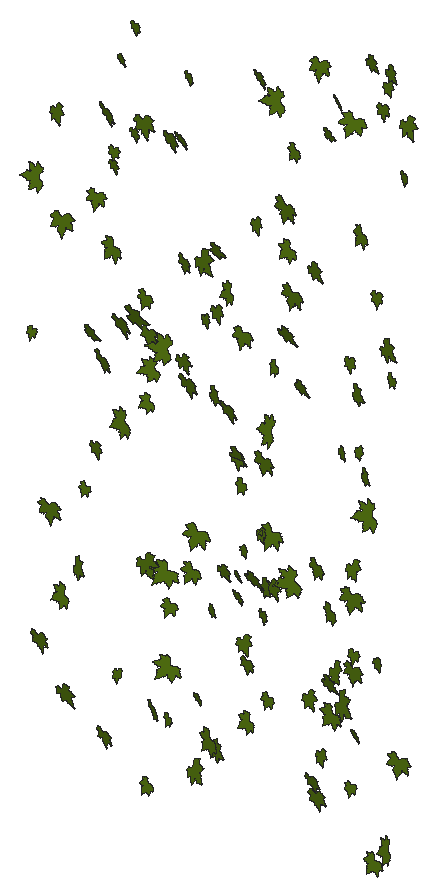
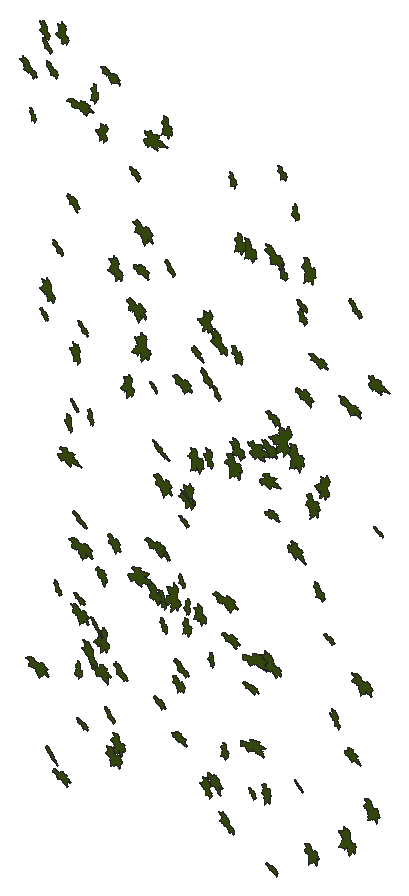
# SketchUp Ruby script. Lengths in inches.
U = 1.inch
M = Sketchup.active_model
def pt(a) = Geom::Point3d.new(a.map { |v| v * U })
def face(e, loops, mat)
  f = e.add_face(loops[0].map { |a| pt(a) })
  loops[1..].each { |l| e.add_face(l.map { |a| pt(a) }).erase! }
  f.material = f.back_material = mat if mat
  f
end
# faces: each face lists its corners as indices into pts; further lists are holes
def faces(e, pts, list, mat = nil) = list.each { |f| face(e, (f[0].is_a?(Array) ? f : [f]).map { |l| l.map { |i| pts[i] } }, mat) }
# xy, xz, yz: faces in a plane at the given z, y or x. An outline is a flat list of corners, or four numbers for a rectangle; further outlines are holes
def ring(l) = l.size == 4 ? [[l[0], l[1]], [l[2], l[1]], [l[2], l[3]], [l[0], l[3]]] : l.each_slice(2).to_a
def flat(e, list, mat, &to3) = list.each { |f| face(e, (f[0].is_a?(Array) ? f : [f]).map { |l| ring(l).map { |u, v| to3.(u, v) } }, mat) }
def xy(e, z, list, mat = nil) = flat(e, list, mat) { |x, y| [x, y, z] }
def xz(e, y, list, mat = nil) = flat(e, list, mat) { |x, z| [x, y, z] }
def yz(e, x, list, mat = nil) = flat(e, list, mat) { |y, z| [x, y, z] }
def lines(e, pts, list) = list.each { |a, b| e.add_line(pt(pts[a]), pt(pts[b])) }
# prism: a flat outline (further loops are holes) pulled along v
def prism(e, loops, v, mat = nil)
  f = face(e, loops, mat); d = Geom::Vector3d.new(v.map { |x| x * U })
  f.pushpull(f.normal.samedirection?(d) ? d.length : -d.length)
end
def box(e, o, s, mat = nil) = prism(e, [[o, [o[0] + s[0], o[1], o[2]], [o[0] + s[0], o[1] + s[1], o[2]], [o[0], o[1] + s[1], o[2]]]], [0, 0, s[2]], mat)
def at(x, y, z, deg = 0) = Geom::Transformation.translation(pt([x, y, z])) * Geom::Transformation.rotation(ORIGIN, Z_AXIS, deg.degrees)
def axes(o, x, y, z) = Geom::Transformation.new([*x, 0, *y, 0, *z, 0, *pt(o).to_a, 1])
def part(name) = M.definitions.add(name)
# library, detail: a bought-in or finely detailed component or shape, given as its bounding box
def library(name, o, s) = part(name).tap { |d| box(d.entities, o, s) }
def detail(e, o, s) = box(e.add_group.entities, o, s)
def put(e, d, t, mat = nil) = e.add_instance(d, t).tap { |i| i.material = mat if mat }
def group(e, t, mat = nil) = e.add_group.tap { |g| g.transformation = t; g.material = mat if mat }.entities
root = M.entities
M.materials.add("[Vegetation Blur 03]").color = [83, 114, 18]
c1 = part("ivy")
xy(c1.entities,0,[[0.782,0,0.786,0,0.787,0.005,0.789,0.009,0.821,0.072,0.875,0.147,1.001,0.272,1.073,0.331,1.137,0.363,1.178,0.379,1.223,0.384,1.272,0.383,1.311,0.374,1.36,0.355,1.399,0.334,1.491,0.285,1.541,0.244,1.583,0.199,1.617,0.15,1.64,0.128,1.662,0.115,1.717,0.105,1.745,0.093,1.784,0.054,1.819,0.057,1.854,0.064,1.882,0.075,1.896,0.074,1.91,0.071,1.937,0.063,1.964,0.053,1.99,0.038,2.016,0.015,2.034,0.002,2.04,0,2.038,0.003,2.036,0.007,2.033,0.038,2.036,0.068,2.045,0.1,2.055,0.116,2.064,0.123,2.077,0.129,2.088,0.129,2.106,0.132,2.118,0.13,2.179,0.132,2.207,0.133,2.225,0.133,2.242,0.138,2.22,0.162,2.207,0.186,2.206,0.213,2.212,0.236,2.228,0.262,2.247,0.274,2.298,0.283,2.355,0.294,2.37,0.296,2.376,0.295,2.377,0.3,2.377,0.303,2.385,0.329,2.411,0.37,2.426,0.392,2.449,0.407,2.511,0.426,2.561,0.444,2.619,0.466,2.589,0.469,2.561,0.476,2.501,0.5,2.449,0.516,2.424,0.523,2.401,0.535,2.377,0.556,2.372,0.568,2.36,0.575,2.268,0.586,2.225,0.592,2.207,0.599,2.194,0.61,2.143,0.65,2.13,0.664,2.122,0.682,2.123,0.7,2.13,0.719,2.148,0.75,2.17,0.781,2.195,0.807,2.221,0.828,2.284,0.874,2.291,0.88,2.288,0.887,2.276,0.9,2.267,0.916,2.265,0.933,2.273,0.967,2.292,1.002,2.313,1.03,2.334,1.054,2.348,1.067,2.358,1.074,2.363,1.076,2.362,1.081,2.35,1.094,2.347,1.11,2.35,1.143,2.359,1.18,2.385,1.254,2.415,1.324,2.448,1.393,2.45,1.4,2.446,1.398,2.44,1.394,2.427,1.383,2.402,1.36,2.376,1.339,2.345,1.324,2.305,1.309,2.282,1.303,2.273,1.306,2.245,1.294,2.212,1.287,2.187,1.291,2.163,1.301,2.142,1.316,2.134,1.327,2.124,1.325,2.09,1.292,2.053,1.259,2.014,1.234,1.973,1.215,1.954,1.21,1.931,1.208,1.909,1.212,1.893,1.22,1.879,1.233,1.872,1.248,1.867,1.281,1.864,1.319,1.821,1.258,1.773,1.197,1.726,1.141,1.698,1.121,1.679,1.116,1.666,1.117,1.647,1.122,1.632,1.129,1.62,1.141,1.617,1.154,1.617,1.219,1.621,1.254,1.623,1.268,1.623,1.281,1.618,1.314,1.606,1.346,1.603,1.375,1.607,1.403,1.603,1.467,1.599,1.499,1.605,1.525,1.614,1.552,1.629,1.577,1.635,1.589,1.629,1.587,1.618,1.582,1.596,1.566,1.581,1.556,1.568,1.552,1.557,1.55,1.545,1.553,1.531,1.562,1.522,1.572,1.504,1.591,1.486,1.611,1.474,1.631,1.457,1.666,1.455,1.684,1.457,1.698,1.452,1.715,1.444,1.728,1.424,1.754,1.419,1.772,1.423,1.786,1.434,1.819,1.444,1.848,1.446,1.855,1.44,1.861,1.43,1.867,1.386,1.904,1.349,1.948,1.326,1.973,1.31,1.995,1.288,2.048,1.284,2.153,1.287,2.254,1.284,2.255,1.282,2.253,1.278,2.247,1.274,2.237,1.266,2.216,1.226,2.125,1.208,2.076,1.184,2.033,1.155,1.984,1.135,1.942,1.111,1.899,1.083,1.861,1.053,1.85,1.059,1.83,1.061,1.809,1.056,1.79,1.049,1.767,1.04,1.749,1.018,1.733,0.994,1.726,0.942,1.734,0.95,1.6875,0.944,1.645,0.932,1.608,0.911,1.585,0.881,1.58,0.854,1.582,0.828,1.588,0.785,1.618,0.773,1.625,0.775,1.614,0.779,1.598,0.796,1.502,0.818,1.402,0.861,1.283,0.882,1.224,0.894,1.174,0.892,1.148,0.886,1.123,0.881,1.107,0.872,1.099,0.849,1.094,0.818,1.092,0.789,1.098,0.762,1.107,0.753,1.113,0.721,1.139,0.698,1.163,0.678,1.194,0.665,1.224,0.628,1.28,0.612,1.312,0.606,1.327,0.606,1.314,0.599,1.282,0.594,1.267,0.581,1.256,0.544,1.245,0.512,1.244,0.473,1.249,0.444,1.256,0.382,1.288,0.339,1.306,0.324,1.316,0.317,1.324,0.309,1.326,0.27,1.314,0.227,1.313,0.185,1.3125,0.152,1.317,0.122,1.328,0.092,1.345,0.073,1.353,0.079,1.338,0.092,1.308,0.117,1.249,0.13,1.215,0.139,1.164,0.147,1.148,0.157,1.136,0.163,1.122,0.174,1.086,0.177,1.067,0.182,1.054,0.186,1.043,0.191,1.038,0.211,1.028,0.237,1.005,0.25,0.974,0.253,0.96,0.25,0.944,0.242,0.914,0.243,0.906,0.249,0.902,0.26,0.894,0.289,0.88,0.307,0.873,0.322,0.862,0.364,0.799,0.403,0.738,0.431,0.709,0.439,0.691,0.441,0.678,0.4375,0.66,0.428,0.645,0.394,0.623,0.303,0.594,0.255,0.581,0.214,0.577,0.179,0.573,0.173,0.568,0.175,0.561,0.167,0.55,0.141,0.523,0.113,0.503,0.077,0.49,0.045,0.486,0.026,0.485,0.019,0.486,0.011,0.483,0,0.471,0.014,0.467,0.044,0.455,0.058,0.447,0.07,0.438,0.097,0.411,0.125,0.394,0.158,0.377,0.174,0.366,0.182,0.359,0.185,0.361,0.242,0.331,0.253,0.316,0.258,0.303,0.262,0.283,0.274,0.278,0.308,0.274,0.341,0.252,0.366,0.226,0.366,0.222,0.37,0.22,0.38,0.221,0.395,0.221,0.425,0.216,0.45,0.207,0.465,0.192,0.473,0.178,0.484,0.15,0.489,0.116,0.483,0.089,0.468,0.058,0.45,0.035,0.435,0.018,0.429,0.011,0.434,0.012,0.438,0.014,0.469,0.019,0.542,0.016,0.581,0.015,0.612,0.027,0.68,0.055,0.696,0.057,0.712,0.052,0.73,0.045,0.741,0.036,0.766,0.014]])
put(root,c1,axes([28.89,173.7,27.51],[0.18332,-0.13201,0.23981],[0.28131,-0.17522,-0.15841],[-0.10639,-0.6908,-0.00565]),"[Vegetation Blur 03]")
put(root,c1,axes([24.48,173.7,22.26],[0.59751,-0.1415,-0.08723],[-0.11552,-0.16395,-0.48523],[-0.05298,-1.23827,0.07421]),"[Vegetation Blur 03]")
put(root,c1,axes([30.97,173.7,25.6875],[0.30037,-0.23448,-0.48095],[-0.59958,-0.05449,-0.24524],[-0.02777,-1.36002,0.09275]),"[Vegetation Blur 03]")
put(root,c1,axes([14.65,173.7,41.15],[0.5598,-0.34639,0.09978],[0.13771,0.07562,-0.47332],[-0.15594,-1.17668,-0.05979]),"[Vegetation Blur 03]")
put(root,c1,axes([11.74,173.7,39.72],[0.34108,-0.07651,0.26436],[0.30846,-0.23678,-0.27587],[-0.10562,-0.93855,0.04805]),"[Vegetation Blur 03]")
put(root,c1,axes([32.59,173.7,43.74],[0.30667,-0.21087,0.08542],[0.09735,-0.07998,-0.26385],[-0.10945,-0.662,0.00467]),"[Vegetation Blur 03]")
put(root,c1,axes([23.32,173.7,18.92],[0.32867,-0.28906,0.36046],[0.45664,0.0115,-0.27589],[-0.07923,-1.13284,-0.09478]),"[Vegetation Blur 03]")
put(root,c1,axes([31.88,173.7,8.15],[0.33567,-0.36714,-0.32626],[-0.40941,0.10373,-0.29893],[-0.15499,-1.06915,0.08303]),"[Vegetation Blur 03]")
put(root,c1,axes([23.83,173.7,46.01],[0.40968,-0.27629,0.16507],[0.21084,0.00024,-0.34848],[-0.12034,-0.94019,-0.0486]),"[Vegetation Blur 03]")
put(root,c1,axes([13.91,173.7,28.49],[0.13916,-0.21976,0.37305],[0.46529,-0.06512,-0.12164],[-0.06205,-0.98109,-0.07549]),"[Vegetation Blur 03]")
put(root,c1,axes([30.85,173.7,36.73],[0.36627,-0.13941,0.12421],[0.13945,-0.15724,-0.30166],[-0.09113,-0.8009,0.0376]),"[Vegetation Blur 03]")
put(root,c1,axes([17.4,173.7,6.27],[0.36884,-0.18268,-0.08765],[-0.12074,-0.10682,-0.30338],[-0.06956,-0.78327,0.06182]),"[Vegetation Blur 03]")
put(root,c1,axes([15.55,173.7,11.24],[0.27201,-0.08351,0.1346],[0.14493,-0.22002,-0.21655],[-0.08857,-0.61651,0.05905]),"[Vegetation Blur 03]")
put(root,c1,axes([28.28,173.7,15.51],[0.22572,0.02556,0.3673],[0.42622,-0.34586,-0.17068],[-0.14503,-0.97663,0.07006]),"[Vegetation Blur 03]")
put(root,c1,axes([12.04,173.7,9.01],[0.44693,-0.21309,0.34937],[0.42945,-0.06761,-0.37241],[-0.09772,-1.27172,-0.03874]),"[Vegetation Blur 03]")
put(root,c1,axes([30.04,173.7,40.08],[0.46163,-0.2581,-0.13642],[-0.17424,-0.01487,-0.3883],[-0.11538,-1.01019,0.04057]),"[Vegetation Blur 03]")
put(root,c1,axes([30.25,173.7,26.5625],[0.11578,-0.07742,0.31422],[0.36947,-0.22297,-0.09932],[-0.11465,-0.79672,-0.00274]),"[Vegetation Blur 03]")
put(root,c1,axes([21.27,173.7,32.5],[0.35673,-0.12377,0.22075],[0.25958,-0.16822,-0.29423],[-0.09696,-0.90576,0.02448]),"[Vegetation Blur 03]")
put(root,c1,axes([11.84,173.7,34.33],[0.60257,-0.08021,0.1387],[0.16152,-0.21723,-0.48713],[-0.06569,-1.26991,0.07457]),"[Vegetation Blur 03]")
put(root,c1,axes([22.43,173.7,24.94],[0.20255,-0.18759,0.41357],[0.50926,-0.09194,-0.17269],[-0.07578,-1.11921,-0.05513]),"[Vegetation Blur 03]")
put(root,c1,axes([16.46,173.7,30.02],[0.0827,-0.23642,0.52033],[0.64705,-0.03418,-0.07095],[-0.03151,-1.3225,-0.09118]),"[Vegetation Blur 03]")
put(root,c1,axes([25.04,173.7,31.12],[0.30532,-0.22387,-0.07925],[-0.10993,-0.04866,-0.26046],[-0.09582,-0.65751,0.04626]),"[Vegetation Blur 03]")
put(root,c1,axes([23.67,173.7,37.91],[0.28926,-0.09005,0.2261],[0.2622,-0.20395,-0.23621],[-0.09958,-0.79857,0.03483]),"[Vegetation Blur 03]")
put(root,c1,axes([23,173.7,24.12],[0.34373,-0.18323,-0.04475],[-0.06771,-0.09451,-0.28552],[-0.07969,-0.71,0.04955]),"[Vegetation Blur 03]")
put(root,c1,axes([14.1,173.7,22.84],[0.37427,-0.16845,0.18276],[0.21743,-0.11081,-0.31265],[-0.09784,-0.89065,0.00433]),"[Vegetation Blur 03]")
put(root,c1,axes([27.89,173.7,14.87],[0.2552,-0.21443,0.36363],[0.45118,-0.05704,-0.2162],[-0.07626,-1.05507,-0.06222]),"[Vegetation Blur 03]")
put(root,c1,axes([24.18,173.7,17.51],[0.3306,-0.20851,0.08999],[0.10594,-0.063,-0.2822],[-0.10584,-0.71438,-0.00138]),"[Vegetation Blur 03]")
put(root,c1,axes([19.09,173.7,30.18],[0.08303,-0.1967,-0.5076],[-0.62878,-0.07669,-0.06383],[0.02474,-1.28895,0.08126]),"[Vegetation Blur 03]")
put(root,c1,axes([19.4,173.7,34.79],[0.45964,-0.254,0.03008],[0.03689,-0.00973,-0.3884],[-0.12342,-0.94883,-0.00407]),"[Vegetation Blur 03]")
put(root,c1,axes([21.01,173.7,10.22],[0.52518,-0.29878,-0.23016],[-0.2856,0.04291,-0.44284],[-0.13799,-1.22592,0.0406]),"[Vegetation Blur 03]")
put(root,c1,axes([16.68,173.7,41.1],[0.56013,-0.13091,0.22183],[0.26451,-0.15182,-0.45897],[-0.08921,-1.27215,0.03195]),"[Vegetation Blur 03]")
put(root,c1,axes([30.47,173.7,48.75],[0.24867,-0.15858,0.33537],[0.40835,-0.11898,-0.21053],[-0.08971,-0.98119,-0.02867]),"[Vegetation Blur 03]")
put(root,c1,axes([22.74,173.7,18.86],[0.1642,-0.18374,0.20113],[0.24769,-0.08699,-0.14719],[-0.08574,-0.60314,-0.04004]),"[Vegetation Blur 03]")
put(root,c1,axes([28.57,173.7,46.38],[0.3403,-0.29163,0.09942],[0.13762,0.03874,-0.29588],[-0.12643,-0.74278,-0.05447]),"[Vegetation Blur 03]")
put(root,c1,axes([27.5,173.7,11.01],[0.30019,-0.07683,0.21744],[0.25164,-0.21034,-0.24309],[-0.09515,-0.7987,0.0431]),"[Vegetation Blur 03]")
put(root,c1,axes([18.42,173.7,40.88],[0.47833,-0.24749,0.17674],[0.22101,-0.01127,-0.40089],[-0.11188,-1.08043,-0.0363]),"[Vegetation Blur 03]")
put(root,c1,axes([30.72,173.7,6.99],[0.48428,-0.17048,-0.13656],[-0.17611,-0.0992,-0.39652],[-0.06201,-1.04969,0.05965]),"[Vegetation Blur 03]")
put(root,c1,axes([29.26,173.7,32.67],[0.3385,-0.12078,0.12895],[0.14584,-0.15588,-0.27795],[-0.08451,-0.75275,0.03687]),"[Vegetation Blur 03]")
put(root,c1,axes([19.98,173.7,20.72],[0.62885,-0.10059,-0.07918],[-0.103,-0.17922,-0.50906],[-0.03454,-1.29703,0.07648]),"[Vegetation Blur 03]")
put(root,c1,axes([24.46,173.7,18.98],[0.40007,-0.13518,0.27607],[0.33165,-0.13835,-0.33079],[-0.0935,-1.06919,0.0079]),"[Vegetation Blur 03]")
put(root,c1,axes([24.23,173.7,18.53],[0.13511,-0.04438,0.35866],[0.42367,-0.24214,-0.11102],[-0.11873,-0.91459,0.01199]),"[Vegetation Blur 03]")
put(root,c1,axes([26.28,173.7,30.07],[0.25746,-0.20708,0.31713],[0.39391,-0.05224,-0.21837],[-0.07715,-0.95777,-0.05666]),"[Vegetation Blur 03]")
put(root,c1,axes([15.25,173.7,34.3],[0.50454,-0.20666,-0.19788],[-0.2502,-0.0525,-0.4163],[-0.0792,-1.15072,0.05453]),"[Vegetation Blur 03]")
put(root,c1,axes([26.98,173.7,36.5],[0.30631,-0.15054,0.36025],[0.43855,-0.11732,-0.25607],[-0.08874,-1.09937,-0.022]),"[Vegetation Blur 03]")
put(root,c1,axes([27.25,173.7,47.9375],[0.54024,-0.08088,0.09089],[0.10321,-0.19815,-0.43637],[-0.05739,-1.11765,0.07079]),"[Vegetation Blur 03]")
put(root,c1,axes([15.36,173.7,30.11],[0.57292,-0.29787,0.17247],[0.22282,0.05394,-0.47834],[-0.12636,-1.25544,-0.06147]),"[Vegetation Blur 03]")
put(root,c1,axes([28.6,173.7,13.62],[0.16056,0.04012,0.53459],[0.63688,-0.33645,-0.12344],[-0.15436,-1.34643,0.04677]),"[Vegetation Blur 03]")
put(root,c1,axes([27.27,173.7,21.41],[0.49502,-0.2424,-0.04719],[-0.06027,-0.00753,-0.41504],[-0.11656,-1.02555,0.0142]),"[Vegetation Blur 03]")
put(root,c1,axes([25.19,173.7,39.95],[0.66254,-0.24066,-0.04091],[-0.05165,-0.00895,-0.54898],[-0.11628,-1.36725,0.01079]),"[Vegetation Blur 03]")
put(root,c1,axes([22.51,173.7,25.33],[0.43109,-0.16307,0.09857],[0.11374,-0.09903,-0.3571],[-0.08905,-0.91592,0.02106]),"[Vegetation Blur 03]")
put(root,c1,axes([31.64,173.7,48.58],[0.22749,-0.09368,0.31124],[0.37139,-0.17878,-0.18927],[-0.09787,-0.89612,0.00522]),"[Vegetation Blur 03]")
put(root,c1,axes([19.88,173.7,18.61],[0.48596,-0.138,-0.11802],[-0.15256,-0.12597,-0.39525],[-0.04619,-1.03571,0.0638]),"[Vegetation Blur 03]")
put(root,c1,axes([26.28,173.7,20.5],[0.32603,-0.13943,-0.47145],[-0.58131,-0.12239,-0.26207],[0.01889,-1.35947,0.07195]),"[Vegetation Blur 03]")
put(root,c1,axes([29.61,173.7,12.93],[0.26661,-0.22568,0.1584],[0.20153,-0.02212,-0.2309],[-0.09528,-0.67823,-0.04518]),"[Vegetation Blur 03]")
put(root,c1,axes([20.76,173.7,31.85],[0.25768,-0.12141,0.16925],[0.19637,-0.14245,-0.21521],[-0.08903,-0.66558,0.01519]),"[Vegetation Blur 03]")
put(root,c1,axes([21.27,173.7,27.65],[0.09017,-0.06413,0.35822],[0.42718,-0.20848,-0.07749],[-0.10559,-0.89821,-0.00759]),"[Vegetation Blur 03]")
put(root,c1,axes([25.16,173.7,28.09],[0.21833,-0.37386,-0.44692],[-0.55988,0.15366,-0.2024],[-0.13932,-1.20335,0.113]),"[Vegetation Blur 03]")
put(root,c1,axes([17.14,173.7,32.09],[0.442,-0.16404,-0.03453],[-0.05057,-0.08968,-0.36412],[-0.07475,-0.90929,0.04214]),"[Vegetation Blur 03]")
put(root,c1,axes([18.36,173.7,18.2],[0.52837,-0.04737,-0.26503],[-0.32337,-0.22367,-0.42312],[0.03764,-1.25647,0.08531]),"[Vegetation Blur 03]")
put(root,c1,axes([25.2,173.7,32.62],[0.38193,-0.25872,0.35613],[0.44798,0.02235,-0.31745],[-0.07443,-1.19311,-0.08317]),"[Vegetation Blur 03]")
put(root,c1,axes([30.92,173.7,17.14],[0.25479,-0.12423,0.18023],[0.21133,-0.13383,-0.2135],[-0.08804,-0.68079,0.00908]),"[Vegetation Blur 03]")
put(root,c1,axes([31.16,173.7,46.8],[0.3823,-0.12513,0.1329],[0.15394,-0.13225,-0.31454],[-0.08072,-0.8448,0.02956]),"[Vegetation Blur 03]")
put(root,c1,axes([25.8,173.7,37.8],[0.41213,-0.1677,-0.21359],[-0.27008,-0.08234,-0.33694],[-0.04682,-1.00125,0.06348]),"[Vegetation Blur 03]")
put(root,c1,axes([10.57,173.7,11.66],[0.54065,-0.21536,0.14176],[0.17436,-0.02611,-0.44914],[-0.10356,-1.16826,-0.01609]),"[Vegetation Blur 03]")
put(root,c1,axes([23.48,173.7,11.9],[0.35443,-0.19304,-0.2419],[-0.30587,-0.0509,-0.29211],[-0.05567,-0.94941,0.06485]),"[Vegetation Blur 03]")
put(root,c1,axes([29.75,173.7,30.59],[0.06006,-0.04189,0.40073],[0.47866,-0.22553,-0.0515],[-0.11129,-0.99263,-0.00521]),"[Vegetation Blur 03]")
put(root,c1,axes([32.43,173.7,46.17],[0.38148,-0.02964,0.33346],[0.3977,-0.23961,-0.3064],[-0.09475,-1.12505,0.05647]),"[Vegetation Blur 03]")
put(root,c1,axes([20.25,173.7,34.52],[0.31957,-0.02324,0.46113],[0.55443,-0.24575,-0.25788],[-0.10943,-1.31297,0.04011]),"[Vegetation Blur 03]")
put(root,c1,axes([25.6,173.7,45.66],[0.17867,-0.14742,-0.47769],[-0.58909,-0.10072,-0.14187],[0.02629,-1.25528,0.06748]),"[Vegetation Blur 03]")
put(root,c1,axes([21.79,173.7,27.72],[0.52923,-0.27231,0.14829],[0.19148,0.04522,-0.44212],[-0.11773,-1.15056,-0.05247]),"[Vegetation Blur 03]")
put(root,c1,axes([18.55,173.7,13.21],[0.5099,-0.05447,-0.26558],[-0.32487,-0.20771,-0.40876],[0.03235,-1.22728,0.08097]),"[Vegetation Blur 03]")
put(root,c1,axes([19.76,173.7,44.57],[0.32682,-0.209,0.08086],[0.0994,-0.02803,-0.27901],[-0.10124,-0.70219,-0.01293]),"[Vegetation Blur 03]")
put(root,c1,axes([31.31,173.7,33.63],[0.21618,-0.06557,0.43271],[0.52184,-0.19331,-0.17826],[-0.09899,-1.16227,0.00524]),"[Vegetation Blur 03]")
put(root,c1,axes([10.53,173.7,27.76],[0.29106,-0.10296,0.03164],[0.02588,-0.14904,-0.23485],[-0.05776,-0.58557,0.05421]),"[Vegetation Blur 03]")
put(root,c1,axes([26.82,173.7,9.71],[0.48095,-0.24511,0.14889],[0.18901,0.01686,-0.4023],[-0.10837,-1.05836,-0.04089]),"[Vegetation Blur 03]")
put(root,c1,axes([28.19,173.7,19.37],[0.45232,-0.27078,-0.13351],[-0.16346,0.04761,-0.38403],[-0.13176,-0.98864,0.01808]),"[Vegetation Blur 03]")
put(root,c1,axes([31.9,173.7,32.8125],[0.32645,-0.19251,-0.02516],[-0.03795,-0.04316,-0.27603],[-0.0909,-0.67338,0.02489]),"[Vegetation Blur 03]")
put(root,c1,axes([26.11,173.7,43.04],[0.38208,-0.19358,-0.10183],[-0.13229,-0.03969,-0.31874],[-0.08317,-0.82615,0.03917]),"[Vegetation Blur 03]")
put(root,c1,axes([13.7,173.7,20.64],[0.31975,-0.13436,-0.03342],[-0.05173,-0.10756,-0.26163],[-0.05713,-0.65457,0.04985]),"[Vegetation Blur 03]")
put(root,c1,axes([15.75,173.7,43.92],[0.22551,-0.17157,0.19026],[0.23404,-0.06401,-0.19384],[-0.08079,-0.66437,-0.03046]),"[Vegetation Blur 03]")
put(root,c1,axes([29.86,173.7,27.97],[0.2323,-0.07315,0.16912],[0.19295,-0.17827,-0.18866],[-0.08352,-0.61528,0.03456]),"[Vegetation Blur 03]")
put(root,c1,axes([18.58,173.7,16.16],[0.41492,-0.08686,-0.03354],[-0.04844,-0.1605,-0.33372],[-0.03354,-0.84286,0.067]),"[Vegetation Blur 03]")
put(root,c1,axes([12.58,173.7,14.86],[0.33179,-0.22508,-0.3253],[-0.40723,0.00189,-0.27687],[-0.0707,-1.0672,0.06812]),"[Vegetation Blur 03]")
put(root,c1,axes([29.22,173.7,16.54],[0.56428,-0.16916,0.04285],[0.04868,-0.06133,-0.46503],[-0.08453,-1.16458,0.01826]),"[Vegetation Blur 03]")
put(root,c1,axes([29.27,173.7,45.82],[0.58164,-0.02914,-0.08506],[-0.10504,-0.22356,-0.46637],[0.00547,-1.19524,0.0893]),"[Vegetation Blur 03]")
put(root,c1,axes([19.16,173.7,29.14],[0.40671,-0.14437,0.24599],[0.29835,-0.08915,-0.33679],[-0.0822,-1.03788,-0.00529]),"[Vegetation Blur 03]")
put(root,c1,axes([21.21,173.7,16.33],[0.10915,-0.09215,0.23401],[0.27778,-0.14927,-0.09555],[-0.08399,-0.61343,-0.0119]),"[Vegetation Blur 03]")
put(root,c1,axes([17.98,173.7,28.7],[0.25465,-0.11048,-0.36792],[-0.45313,-0.12762,-0.20287],[0.02807,-1.05778,0.0629]),"[Vegetation Blur 03]")
put(root,c1,axes([24.46,173.7,13.24],[0.37736,-0.14693,-0.03133],[-0.04655,-0.08489,-0.31089],[-0.06637,-0.77592,0.03994]),"[Vegetation Blur 03]")
put(root,c1,axes([21.375,173.7,35.4],[0.10455,-0.16948,0.36645],[0.45413,-0.0579,-0.09052],[-0.04648,-0.94693,-0.06005]),"[Vegetation Blur 03]")
put(root,c1,axes([29.34,173.7,10.16],[0.34421,-0.10508,0.04416],[0.04441,-0.1326,-0.28022],[-0.05969,-0.70465,0.04615]),"[Vegetation Blur 03]")
put(root,c1,axes([11.36,173.7,36.65],[0.1603,-0.20672,-0.46475],[-0.57787,-0.01388,-0.13179],[-0.02063,-1.21728,0.08043]),"[Vegetation Blur 03]")
put(root,c1,axes([19.34,173.7,28.36],[0.58972,-0.25941,0.10506],[0.13617,0.04808,-0.49046],[-0.11798,-1.24117,-0.04096]),"[Vegetation Blur 03]")
put(root,c1,axes([15.25,173.7,38.21],[0.29872,-0.15455,0.15212],[0.18312,-0.07365,-0.25129],[-0.08276,-0.72081,-0.00694]),"[Vegetation Blur 03]")
put(root,c1,axes([22.46,173.7,34.34],[0.30417,-0.25351,-0.27604],[-0.3464,0.04167,-0.26026],[-0.0979,-0.93513,0.06323]),"[Vegetation Blur 03]")
put(root,c1,axes([21.33,173.7,8.72],[0.09186,-0.01547,0.40746],[0.48625,-0.23456,-0.07442],[-0.11344,-1.01793,0.01096]),"[Vegetation Blur 03]")
put(root,c1,axes([31.52,173.7,47.92],[0.26564,-0.06538,0.20861],[0.24422,-0.17627,-0.21582],[-0.08188,-0.73784,0.03307]),"[Vegetation Blur 03]")
put(root,c1,axes([14.5,173.7,7.93],[0.51714,-0.23527,0.06533],[0.0842,0.02179,-0.43163],[-0.1113,-1.07662,-0.02301]),"[Vegetation Blur 03]")
put(root,c1,axes([17.18,173.7,30.17],[0.49069,-0.15556,0.05335],[0.06086,-0.06942,-0.40473],[-0.07927,-1.0163,0.01948]),"[Vegetation Blur 03]")
put(root,c1,axes([14.05,173.7,36.3125],[0.49447,-0.06651,0.04707],[0.05156,-0.17262,-0.39913],[-0.04138,-1.00977,0.06513]),"[Vegetation Blur 03]")
put(root,c1,axes([17.57,173.7,10.47],[0.46353,-0.32199,-0.04056],[-0.03174,0.12476,-0.39742],[-0.16108,-0.95117,-0.0384]),"[Vegetation Blur 03]")
put(root,c1,axes([14.42,173.7,27.97],[0.56984,-0.3114,0.00181],[0.01697,0.11385,-0.47886],[-0.15039,-1.16708,-0.04719]),"[Vegetation Blur 03]")
put(root,c1,axes([25.62,173.7,35.42],[0.63233,-0.20373,-0.05495],[-0.06893,-0.01048,-0.5222],[-0.0979,-1.30853,0.01274]),"[Vegetation Blur 03]")
put(root,c1,axes([27.03,173.7,8.97],[0.52242,-0.17809,0.13316],[0.16214,-0.04009,-0.43214],[-0.08844,-1.12553,-0.00568]),"[Vegetation Blur 03]")
put(root,c1,axes([23.03,173.7,20.32],[0.21446,-0.11197,0.17329],[0.20462,-0.11686,-0.18055],[-0.07858,-0.60992,0.00278]),"[Vegetation Blur 03]")
put(root,c1,axes([31.86,173.7,12.68],[0.62343,-0.11777,0.0104],[0.0079,-0.1089,-0.50918],[-0.0581,-1.27854,0.04241]),"[Vegetation Blur 03]")
put(root,c1,axes([28.11,173.7,43.92],[0.06833,-0.14193,0.31087],[0.38368,-0.0807,-0.06197],[-0.05132,-0.79223,-0.04938]),"[Vegetation Blur 03]")
put(root,c1,axes([22.59,173.7,17.92],[0.34195,-0.22556,0.12659],[0.16367,0.01646,-0.28987],[-0.09636,-0.7725,-0.04314]),"[Vegetation Blur 03]")
put(root,c1,axes([16.78,173.7,17.4375],[0.45366,-0.05419,0.38117],[0.46073,-0.18,-0.36926],[-0.08098,-1.3277,0.0345]),"[Vegetation Blur 03]")
put(root,c1,axes([16.48,173.7,40.34],[0.3125,-0.15896,0.12959],[0.15654,-0.05797,-0.26261],[-0.08171,-0.71898,-0.00748]),"[Vegetation Blur 03]")
put(root,c1,axes([24.01,173.7,21.52],[0.23635,-0.06465,0.19523],[0.22776,-0.16748,-0.19239],[-0.07957,-0.67142,0.02919]),"[Vegetation Blur 03]")
put(root,c1,axes([18.65,173.7,10.1],[0.29646,-0.18293,-0.03481],[-0.04858,-0.02904,-0.25162],[-0.08579,-0.61566,0.02221]),"[Vegetation Blur 03]")
put(root,c1,axes([16.15,173.7,25.4375],[0.39569,-0.25539,-0.40505],[-0.50198,0.05522,-0.33211],[-0.09868,-1.305,0.06522]),"[Vegetation Blur 03]")
put(root,c1,axes([28.2,173.7,14.03],[0.51915,-0.17766,-0.225],[-0.28069,-0.03421,-0.42714],[-0.06834,-1.20911,0.04515]),"[Vegetation Blur 03]")
put(root,c1,axes([20.25,173.7,11.625],[0.27556,-0.19726,0.13683],[0.17351,-0.01114,-0.23526],[-0.08482,-0.66366,-0.03672]),"[Vegetation Blur 03]")
put(root,c1,axes([29.27,173.7,21.47],[0.29882,0.02623,0.28715],[0.33985,-0.26962,-0.23169],[-0.09199,-0.91085,0.07685]),"[Vegetation Blur 03]")
put(root,c1,axes([22.76,173.7,15.31],[0.35031,-0.0224,0.27157],[0.32357,-0.21117,-0.28075],[-0.0784,-0.97156,0.05476]),"[Vegetation Blur 03]")
put(root,c1,axes([16.56,173.7,46.1],[0.3345,-0.16348,0.07359],[0.08724,-0.0471,-0.28058],[-0.08265,-0.71135,0.00167]),"[Vegetation Blur 03]")
put(root,c1,axes([19.12,173.7,41.0625],[0.39765,-0.2594,0.13842],[0.18466,0.06494,-0.33421],[-0.10274,-0.88724,-0.06493]),"[Vegetation Blur 03]")
put(root,c1,axes([23.08,173.7,14.65],[0.43055,-0.17357,0.04955],[0.0586,-0.03425,-0.35804],[-0.08583,-0.8941,0.0041]),"[Vegetation Blur 03]")
put(root,c1,axes([19.81,173.7,7.21],[0.24806,0.03915,0.43187],[0.51673,-0.28046,-0.19369],[-0.11561,-1.16947,0.06091]),"[Vegetation Blur 03]")
put(root,c1,axes([13.14,173.7,15.54],[0.07106,0.03212,0.39333],[0.4647,-0.27217,-0.05243],[-0.12873,-0.96482,0.02788]),"[Vegetation Blur 03]")
put(root,c1,axes([29.06,173.7,20.47],[0.64834,-0.11558,0.00243],[-0.00125,-0.10055,-0.52962],[-0.05623,-1.33037,0.03982]),"[Vegetation Blur 03]")
put(root,c1,axes([21.64,173.7,18.79],[0.32691,-0.16543,0.24576],[0.30294,-0.04245,-0.2729],[-0.07327,-0.91364,-0.03182]),"[Vegetation Blur 03]")
put(root,c1,axes([23.94,173.7,25.91],[0.59559,-0.20487,-0.02237],[-0.02751,0.00349,-0.49282],[-0.09953,-1.2269,0.00233]),"[Vegetation Blur 03]")
put(root,c1,axes([26.67,173.7,13.6875],[0.31135,-0.03304,0.2876],[0.34314,-0.19604,-0.25097],[-0.08184,-0.94759,0.04189]),"[Vegetation Blur 03]")
put(root,c1,axes([17.59,173.7,26.7],[0.28967,-0.12811,-0.2275],[-0.2852,-0.08534,-0.23432],[-0.01552,-0.82284,0.05972]),"[Vegetation Blur 03]")
put(root,c1,axes([15.29,173.7,39.01],[0.33002,-0.10362,0.05882],[0.06392,-0.11285,-0.27012],[-0.06037,-0.68589,0.03556]),"[Vegetation Blur 03]")
put(root,c1,axes([29.53,173.7,17.28],[0.33589,-0.10606,0.03492],[0.03467,-0.10992,-0.27466],[-0.05731,-0.68805,0.03849]),"[Vegetation Blur 03]")
put(root,c1,axes([11.05,173.7,18.79],[0.61675,-0.12461,0.11294],[0.13479,-0.08629,-0.50526],[-0.06818,-1.29784,0.02275]),"[Vegetation Blur 03]")
put(root,c1,axes([22.73,173.7,32.1],[0.54066,-0.11979,-0.01485],[-0.02304,-0.09186,-0.44216],[-0.05647,-1.10941,0.03821]),"[Vegetation Blur 03]")
